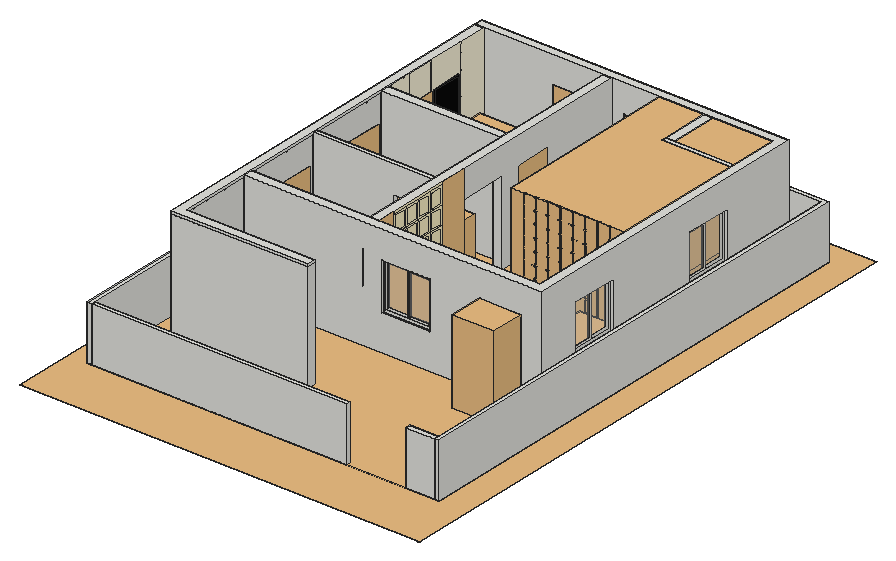
# SketchUp Ruby script. Lengths in inches.
U = 1.inch
M = Sketchup.active_model
def pt(a) = Geom::Point3d.new(a.map { |v| v * U })
def face(e, loops, mat)
  f = e.add_face(loops[0].map { |a| pt(a) })
  loops[1..].each { |l| e.add_face(l.map { |a| pt(a) }).erase! }
  f.material = f.back_material = mat if mat
  f
end
# faces: each face lists its corners as indices into pts; further lists are holes
def faces(e, pts, list, mat = nil) = list.each { |f| face(e, (f[0].is_a?(Array) ? f : [f]).map { |l| l.map { |i| pts[i] } }, mat) }
# xy, xz, yz: faces in a plane at the given z, y or x. An outline is a flat list of corners, or four numbers for a rectangle; further outlines are holes
def ring(l) = l.size == 4 ? [[l[0], l[1]], [l[2], l[1]], [l[2], l[3]], [l[0], l[3]]] : l.each_slice(2).to_a
def flat(e, list, mat, &to3) = list.each { |f| face(e, (f[0].is_a?(Array) ? f : [f]).map { |l| ring(l).map { |u, v| to3.(u, v) } }, mat) }
def xy(e, z, list, mat = nil) = flat(e, list, mat) { |x, y| [x, y, z] }
def xz(e, y, list, mat = nil) = flat(e, list, mat) { |x, z| [x, y, z] }
def yz(e, x, list, mat = nil) = flat(e, list, mat) { |y, z| [x, y, z] }
def lines(e, pts, list) = list.each { |a, b| e.add_line(pt(pts[a]), pt(pts[b])) }
# prism: a flat outline (further loops are holes) pulled along v
def prism(e, loops, v, mat = nil)
  f = face(e, loops, mat); d = Geom::Vector3d.new(v.map { |x| x * U })
  f.pushpull(f.normal.samedirection?(d) ? d.length : -d.length)
end
def box(e, o, s, mat = nil) = prism(e, [[o, [o[0] + s[0], o[1], o[2]], [o[0] + s[0], o[1] + s[1], o[2]], [o[0], o[1] + s[1], o[2]]]], [0, 0, s[2]], mat)
def at(x, y, z, deg = 0) = Geom::Transformation.translation(pt([x, y, z])) * Geom::Transformation.rotation(ORIGIN, Z_AXIS, deg.degrees)
def axes(o, x, y, z) = Geom::Transformation.new([*x, 0, *y, 0, *z, 0, *pt(o).to_a, 1])
def part(name) = M.definitions.add(name)
# library, detail: a bought-in or finely detailed component or shape, given as its bounding box
def library(name, o, s) = part(name).tap { |d| box(d.entities, o, s) }
def detail(e, o, s) = box(e.add_group.entities, o, s)
def put(e, d, t, mat = nil) = e.add_instance(d, t).tap { |i| i.material = mat if mat }
def group(e, t, mat = nil) = e.add_group.tap { |g| g.transformation = t; g.material = mat if mat }.entities
root = M.entities
M.materials.add("0939 AP 7866 BUTTER SCOTCH").color = [249, 239, 196]
M.materials.add("0949 AP 7872 SAFFRON SMILE").color = [254, 228, 149]
M.materials.add("0976 AP 9885 Military Boots-N").color = [124, 94, 57]
M.materials.add("0977 AP 7900 CANDLE LIGHT").color = [247, 240, 215]
M.materials.add("CLC2-EXTRACTOR-Cristal placa").color = [10, 10, 10]
M.materials.add("Cattelan Italy Adam 3").color = [207, 207, 207]
M.materials.add("[Color M00]").color = [255, 255, 255]
M.materials.add("[Color M09]").color = [0, 0, 0]
M.materials.add("[CoolGray4]").color = [225, 226, 230]
M.materials["[CoolGray4]"].alpha = 0.26
M.materials.add("[Translucent Glass Gray]").color = [128, 128, 128]
M.materials["[Translucent Glass Gray]"].alpha = 0.5
M.materials.add("[Translucent Glass Tinted]1").color = [7, 201, 240]
M.materials["[Translucent Glass Tinted]1"].alpha = 0.48
M.materials.add("[Wood Cherry Original]").color = [152, 86, 42]
M.materials.add("[Wood Floor Parquet]").color = [145, 89, 39]
M.materials.add("[Wood Veneer 02]").color = [190, 128, 91]
c1 = library("FLOOPLAN+DWG.dwg",[0,0,0],[402.1875,574.41,0.01])
c2 = part("Window sash")
g1 = group(c2.entities,at(0.98,0,0))
prism(g1,[[[-0.98,0,0],[30.98,0,0],[30.98,0,45.6],[-0.98,0,45.6]],[[29.01,0,43.625],[29.01,0,1.97],[0.98,0,1.97],[0.98,0,43.625]]],[0,1.18,0])
g2 = group(c2.entities,at(1.97,0.59,1.97))
xz(g2,0,[[0,0,28.03,41.66]],"[CoolGray4]")
c3 = part("Sliding window")
put(c3.entities,c2,at(31.97,2.82,1.97))
put(c3.entities,c2,at(1.97,1.25,1.97))
g3 = group(c3.entities,at(0,0,0))
prism(g3,[[[65.9,4.72,0],[0,4.72,0],[0,4.72,49.53],[65.9,4.72,49.53]],[[1.97,4.72,47.5625],[1.97,4.72,1.97],[63.93,4.72,1.97],[63.93,4.72,47.5625]]],[0,-4.72,0])
c4 = part("ventilator")
g4 = group(c4.entities,at(0,0,0))
xy(g4,0,[[0,0,24,1],[0,1,24,6.83]],"[Wood Floor Parquet]")
xy(g4,1.75,[[2,0,22,6.83]],"[Wood Floor Parquet]")
xy(g4,21.87,[[2,0,22,6.83]],"[Wood Cherry Original]")
xy(g4,23.62,[[0,0,24,1],[0,1,24,6.83]],"[Wood Floor Parquet]")
xz(g4,0,[[[0,0,24,23.62],[2,1.75,22,21.87]]],"[Wood Floor Parquet]")
xz(g4,6.83,[[[0,0,24,23.62],[2,1.75,22,21.87]]],"[Wood Cherry Original]")
yz(g4,0,[[0,0,1,23.62],[1,0,6.83,23.62]],"[Wood Floor Parquet]")
yz(g4,2,[[0,1.75,6.83,1.75,6.83,7.66,0,3.5],[0,3.5,6.83,7.66,6.83,11.8125,0,7.66],[0,7.66,6.83,11.8125,6.83,15.97,0,11.8125],[0,11.8125,6.83,15.97,6.83,20.12,0,15.97],[0,15.97,6.83,20.12,6.83,21.87,0,21.87]],"[Wood Floor Parquet]")
yz(g4,22,[[0,1.75,0,3.5,6.83,7.66,6.83,1.75],[0,3.5,0,7.66,6.83,11.8125,6.83,7.66],[0,7.66,0,11.8125,6.83,15.97,6.83,11.8125],[0,11.8125,0,15.97,6.83,20.12,6.83,15.97],[0,15.97,0,21.87,6.83,21.87,6.83,20.12]],"[Wood Floor Parquet]")
yz(g4,24,[[0,0,1,23.62],[1,0,6.83,23.62]],"[Wood Floor Parquet]")
p = [[2,0,3.5],[2,6.83,7.66],[22,6.83,7.66],[22,0,3.5],[2,6.83,11.8125],[2,0,7.66],
  [22,0,7.66],[22,6.83,11.8125],[2,0,11.8125],[2,6.83,15.97],[22,6.83,15.97],[22,0,11.8125],
  [2,6.83,20.12],[2,0,15.97],[22,0,15.97],[22,6.83,20.12]]
faces(g4,p,[[0,1,2,3],[4,5,6,7],[8,9,10,11]],"[Translucent Glass Tinted]1")
faces(g4,p,[[12,13,14,15]],"[Translucent Glass Gray]")
c5 = library("door by lz",[5.91,-4.92,0],[35.43,6.61,78.74])
c6 = library("Open hinged door",[0,0,0],[71.65,72.83,104.72])
c7 = library("Wall hung toilet",[0.42,0,0],[26.94,19.69,42.125])
c8 = library("3D DOOR",[-0.52,0,0],[35.44,5.29,86.61])
c9 = library("DINING SET",[25.27,8.07,0],[68.7,94.48,53.71])
c10 = library("Спалня Венид",[0.07,-0.07,0],[84.71,86.8,39])
c11 = library("window curtain",[0,0,0],[144.39,2.04,43.18])
c12 = library("sofaD71839)",[0.35,-39.08,0.31],[80.46,34.29,30.24])
c13 = library("Layer_AVLA\#1",[-10.99,-0.19,-10.42],[21.98,0.74,15.78])
c14 = part("Group12\#1")
xy(c14.entities,0,[[329.9,217.87,329.9,226.87,341.6,226.87,341.6,519.37,41.6,519.37,41.6,528.37,350.6,528.37,350.6,217.87],[50.6,217.87,287.9,226.87]])
xy(c14.entities,36,[[189.83,217.87,237.83,226.87],[341.6,260,350.6,308],[341.6,403.49,350.6,451.49]])
xy(c14.entities,48,[[123.82,519.37,159.82,528.37]])
xy(c14.entities,60,[[192.32,519.37,216.32,528.37],[300.77,519.37,324.77,528.37]])
xy(c14.entities,84,[[189.83,217.87,237.83,226.87],[287.9,217.87,329.9,226.87],[341.6,260,350.6,308],[341.6,403.49,350.6,451.49],[123.82,519.37,159.82,528.37],
  [192.32,519.37,216.32,528.37],[300.77,519.37,324.77,528.37]])
xy(c14.entities,112,[[50.6,217.87,350.6,217.87,350.6,528.37,41.6,528.37,41.6,519.37,341.6,519.37,341.6,226.87,50.6,226.87]])
xz(c14.entities,217.87,[[[50.6,0,287.9,0,287.9,84,329.9,84,329.9,0,350.6,0,350.6,112,50.6,112],[189.83,36,237.83,84]]])
xz(c14.entities,226.87,[[[50.6,0,50.6,112,341.6,112,341.6,0,329.9,0,329.9,84,287.9,84,287.9,0],[189.83,36,237.83,84]]])
xz(c14.entities,260,[[341.6,36,350.6,84]])
xz(c14.entities,308,[[341.6,36,350.6,84]])
xz(c14.entities,403.49,[[341.6,36,350.6,84]])
xz(c14.entities,451.49,[[341.6,36,350.6,84]])
xz(c14.entities,519.37,[[[41.6,0,341.6,112],[123.82,48,159.82,84],[192.32,60,216.32,84],[300.77,60,324.77,84]]])
xz(c14.entities,528.37,[[[41.6,0,350.6,112],[123.82,48,159.82,84],[192.32,60,216.32,84],[300.77,60,324.77,84]]])
yz(c14.entities,41.6,[[519.37,0,528.37,112]])
yz(c14.entities,50.6,[[217.87,0,226.87,112]])
yz(c14.entities,123.82,[[519.37,48,528.37,84]])
yz(c14.entities,159.82,[[519.37,48,528.37,84]])
yz(c14.entities,189.83,[[217.87,36,226.87,84]])
yz(c14.entities,192.32,[[519.37,60,528.37,84]])
yz(c14.entities,216.32,[[519.37,60,528.37,84]])
yz(c14.entities,237.83,[[217.87,36,226.87,84]])
yz(c14.entities,287.9,[[217.87,0,226.87,84]])
yz(c14.entities,300.77,[[519.37,60,528.37,84]])
yz(c14.entities,324.77,[[519.37,60,528.37,84]])
yz(c14.entities,329.9,[[217.87,0,226.87,84]])
yz(c14.entities,341.6,[[[226.87,0,519.37,112],[260,36,308,84],[403.49,36,451.49,84]]])
yz(c14.entities,350.6,[[[217.87,0,528.37,112],[260,36,308,84],[403.49,36,451.49,84]]])
c15 = part("Group13\#1")
xy(c15.entities,0,[[41.6,136.87,41.6,519.37,50.6,519.37,50.6,491.06,51.07,491.06,51.07,490.59,50.6,490.59,50.6,145.87,179.6,145.87,179.6,136.87],[50.6,399.37,51.07,452.7],[50.6,452.7,51.07,453.17],[50.6,453.17,51.07,490.59],[50.6,491.06,51.07,519.37]])
xy(c15.entities,36,[[41.6,250.14,50.6,298.14],[41.6,336.36,50.6,384.36],[41.6,403.49,50.6,451.49],[50.6,403.49,51.07,451.49]])
xy(c15.entities,84,[[41.6,250.14,50.6,298.14],[41.6,336.36,50.6,384.36],[41.6,403.49,50.6,451.49],[50.6,403.49,51.07,451.49]])
xy(c15.entities,109.4375,[[41.6,136.87,41.6,519.37,50.6,519.37,50.6,145.87,179.6,145.87,179.6,136.87]])
xy(c15.entities,112,[[41.6,136.87,179.6,136.87,179.6,145.87,50.6,145.87,50.6,519.37,41.6,519.37],[50.6,399.37,51.07,452.7],[50.6,452.7,51.07,453.17],[50.6,453.17,51.07,490.59],[50.6,490.59,51.07,491.06],
  [50.6,491.06,51.07,519.37]])
xz(c15.entities,136.87,[[41.6,0,179.6,109.4375],[41.6,109.4375,179.6,112]])
xz(c15.entities,145.87,[[50.6,0,179.6,109.4375],[50.6,109.4375,179.6,112]])
xz(c15.entities,250.14,[[41.6,36,50.6,84]])
xz(c15.entities,298.14,[[41.6,36,50.6,84]])
xz(c15.entities,336.36,[[41.6,36,50.6,84]])
xz(c15.entities,384.36,[[41.6,36,50.6,84]])
xz(c15.entities,399.37,[[50.6,0,51.07,112]])
xz(c15.entities,403.49,[[41.6,36,50.6,84],[50.6,36,51.07,84]])
xz(c15.entities,451.49,[[41.6,36,50.6,84],[50.6,36,51.07,84]])
xz(c15.entities,452.7,[[50.6,0,51.07,112]])
xz(c15.entities,453.17,[[50.6,0,51.07,112]])
xz(c15.entities,490.59,[[50.6,0,51.07,109.4375],[50.6,109.4375,51.07,112]])
xz(c15.entities,491.06,[[50.6,0,51.07,109.4375],[50.6,109.4375,51.07,112]])
xz(c15.entities,519.37,[[41.6,0,50.6,109.4375],[50.6,0,51.07,112],[41.6,109.4375,50.6,112]])
yz(c15.entities,41.6,[[[136.87,0,519.37,109.4375],[250.14,36,298.14,84],[336.36,36,384.36,84],[403.49,36,451.49,84]],[136.87,109.4375,519.37,112]])
yz(c15.entities,50.6,[[[145.87,0,399.37,109.4375],[250.14,36,298.14,84],[336.36,36,384.36,84]],[[399.37,0,452.7,109.4375],[403.49,36,451.49,84]],[452.7,0,453.17,109.4375],[453.17,0,490.59,109.4375],[491.06,0,519.37,109.4375],
  [145.87,109.4375,399.37,112],[399.37,109.4375,452.7,112],[452.7,109.4375,453.17,112],[453.17,109.4375,490.59,112],[490.59,109.4375,491.06,112],
  [491.06,109.4375,519.37,112]])
yz(c15.entities,51.07,[[427.02,0,427.49,36],[452.7,0,453.17,112],[490.59,0,491.06,112],[425.5625,84,426.04,112]],"0976 AP 9885 Military Boots-N")
yz(c15.entities,51.07,[[399.37,0,427.02,0,427.02,36,403.49,36,403.49,84,425.5625,84,425.5625,112,399.37,112],[427.49,0,452.7,0,452.7,112,426.04,112,426.04,84,451.49,84,451.49,36,427.49,36],[453.17,0,490.59,112],[491.06,0,519.37,112]],"0977 AP 7900 CANDLE LIGHT")
yz(c15.entities,179.6,[[136.87,0,145.87,109.4375],[136.87,109.4375,145.87,112]])
c16 = library("Group621\#1",[-13.47,-47,0],[26.94,94,0.5])
c17 = library("Group691\#2",[-8.65,-47,0],[17.3,94,0.5])
c18 = part("Group14\#1")
xy(c18.entities,0,[[170.6,226.87,179.6,333.37],[170.6,381.37,179.6,402.37],[170.6,438.37,179.6,519.37]])
xy(c18.entities,84,[[170.6,333.37,179.6,381.37],[170.6,402.37,179.6,438.37]])
xy(c18.entities,112,[[170.6,226.87,179.6,519.37]])
xz(c18.entities,226.87,[[170.6,0,179.6,112]])
xz(c18.entities,333.37,[[170.6,0,179.6,84]])
xz(c18.entities,381.37,[[170.6,0,179.6,84]])
xz(c18.entities,402.37,[[170.6,0,179.6,84]])
xz(c18.entities,438.37,[[170.6,0,179.6,84]])
xz(c18.entities,519.37,[[170.6,0,179.6,112]])
yz(c18.entities,170.6,[[226.87,0,226.87,112,519.37,112,519.37,0,438.37,0,438.37,84,402.37,84,402.37,0,381.37,0,381.37,84,333.37,84,333.37,0]])
yz(c18.entities,179.6,[[226.87,0,333.37,18],[381.37,0,402.37,0,402.37,84,438.37,84,438.37,0,519.37,0,519.37,112,333.37,112,333.37,84,381.37,84],[244.16,18,244.87,112]])
yz(c18.entities,179.6,[[244.87,18,306.43,112]],"0939 AP 7866 BUTTER SCOTCH")
put(c18.entities,c16,axes([179.6,319.76,65],[0,1,0],[0,0,1],[1,0,0]),"0939 AP 7866 BUTTER SCOTCH")
put(c18.entities,c17,axes([179.6,235.52,65],[0,1,0],[0,0,1],[1,0,0]),"0939 AP 7866 BUTTER SCOTCH")
c19 = part("Group15\#1")
box(c19.entities,[50.6,390.37,0],[120,9,112])
c20 = library("Group16\#1",[227.6,332.87,0],[114,186.5,112])
c21 = part("Group17\#1")
box(c21.entities,[272.6,471.37,0],[9,48,112])
c22 = part("Group18\#1")
prism(c22.entities,[[[341.6,471.37,0],[338.6,471.37,0],[338.6,471.37,84],[312.6,471.37,84],[312.6,471.37,0],[272.6,471.37,0],[272.6,471.37,112],[341.6,471.37,112]]],[0,-4.5,0])
c23 = part("Group19\#1")
prism(c23.entities,[[[170.6,309.37,0],[167.6,309.37,0],[167.6,309.37,84],[131.6,309.37,84],[131.6,309.37,0],[50.6,309.37,0],[50.6,309.37,112],[170.6,309.37,112]]],[0,-4.5,0])
c24 = part("Group26\#1")
box(c24.entities,[340.13,60.37,0],[28.47,4.5,54.875])
c25 = part("Group24\#1")
prism(c25.entities,[[[368.6,546.37,0],[23.6,546.37,0],[23.6,60.37,0],[19.1,60.37,0],[19.1,550.87,0],[373.1,550.87,0],[373.1,60.37,0],[368.6,60.37,0]]],[0,0,54.875])
put(c25.entities,c24,at(0,0,0))
c26 = part("Group25\#1")
box(c26.entities,[23.6,60.37,0],[256.53,4.5,54.875])
c27 = library("Group\#12",[0,-0.0625,0],[48,15.0625,24])
c28 = library("Group\#13",[0,-0.13,0],[120,18.13,42.48])
c29 = library("Group\#14",[0,-8.89,-5.43],[120,21.66,33.43])
c30 = part("Group\#15")
prism(c30.entities,[[[1.2,0.71,0],[0.83,0.71,0.03],[0.53,0.71,0.13],[0.3,0.71,0.3],[0.13,0.71,0.53],[0.03,0.71,0.83],[0,0.71,1.2],[0,0.71,10.8],[0.03,0.71,11.17],[0.13,0.71,11.47],[0.3,0.71,11.7],[0.53,0.71,11.87],[0.83,0.71,11.97],[1.2,0.71,12],[10.8,0.71,12],[11.17,0.71,11.97],[11.47,0.71,11.87],[11.7,0.71,11.7],[11.87,0.71,11.47],[11.97,0.71,11.17],[12,0.71,10.8],[12,0.71,1.2],[11.97,0.71,0.83],[11.87,0.71,0.53],[11.7,0.71,0.3],[11.47,0.71,0.13],[11.17,0.71,0.03],[10.8,0.71,0]]],[0,-0.39,0])
c31 = part("Group\#17")
xy(c31.entities,0,[[0,0,0.47,15]])
xy(c31.entities,1.35,[[0.24,1.82,0.47,13.18]])
xy(c31.entities,16.65,[[0.24,1.82,0.47,13.18]])
xy(c31.entities,18,[[0,0,0.47,15]])
xz(c31.entities,0,[[0,0,0.47,18]])
xz(c31.entities,1.35,[[0.24,1.82,0.47,16.18]])
xz(c31.entities,13.65,[[0.24,1.82,0.47,16.18]])
xz(c31.entities,15,[[0,0,0.47,18]])
yz(c31.entities,0,[[0,0,15,18]])
yz(c31.entities,0.24,[[1.82,1.35,13.18,1.35,13.33,1.36,13.44,1.4,13.54,1.46,13.6,1.56,13.64,1.67,13.65,1.82,13.65,16.18,13.64,16.33,13.6,16.44,13.54,16.54,13.44,16.6,13.33,16.64,13.18,16.65,1.82,16.65,1.67,16.64,1.56,16.6,1.46,16.54,1.4,16.44,1.36,16.33,1.35,16.18,1.35,1.82,1.36,1.67,1.4,1.56,1.46,1.46,1.56,1.4,1.67,1.36]])
yz(c31.entities,0.47,[[[0,0,15,18],[1.82,1.35,1.67,1.36,1.56,1.4,1.46,1.46,1.4,1.56,1.36,1.67,1.35,1.82,1.35,16.18,1.36,16.33,1.4,16.44,1.46,16.54,1.56,16.6,1.67,16.64,1.82,16.65,13.18,16.65,13.33,16.64,13.44,16.6,13.54,16.54,13.6,16.44,13.64,16.33,13.65,16.18,13.65,1.82,13.64,1.67,13.6,1.56,13.54,1.46,13.44,1.4,13.33,1.36,13.18,1.35]]])
p = [[0.47,1.82,1.35],[0.24,1.82,1.35],[0.24,1.67,1.36],[0.47,1.67,1.36],[0.47,13.33,1.36],[0.24,13.33,1.36],
  [0.24,13.18,1.35],[0.47,13.18,1.35],[0.47,1.56,1.4],[0.24,1.56,1.4],[0.24,1.46,1.46],[0.47,1.46,1.46],
  [0.47,13.44,1.4],[0.24,13.44,1.4],[0.47,13.54,1.46],[0.24,13.54,1.46],[0.24,1.4,1.56],[0.47,1.4,1.56],
  [0.47,13.6,1.56],[0.24,13.6,1.56],[0.24,1.36,1.67],[0.47,1.36,1.67],[0.47,13.64,1.67],[0.24,13.64,1.67],
  [0.24,1.35,1.82],[0.47,1.35,1.82],[0.47,13.65,1.82],[0.24,13.65,1.82],[0.24,1.36,16.33],[0.47,1.36,16.33],
  [0.47,1.35,16.18],[0.24,1.35,16.18],[0.47,13.64,16.33],[0.24,13.64,16.33],[0.24,13.65,16.18],[0.47,13.65,16.18],
  [0.24,1.4,16.44],[0.47,1.4,16.44],[0.47,13.6,16.44],[0.24,13.6,16.44],[0.24,1.46,16.54],[0.47,1.46,16.54],
  [0.47,13.54,16.54],[0.24,13.54,16.54],[0.24,1.56,16.6],[0.47,1.56,16.6],[0.47,13.44,16.6],[0.24,13.44,16.6],
  [0.24,1.67,16.64],[0.47,1.67,16.64],[0.24,1.82,16.65],[0.47,1.82,16.65],[0.47,13.18,16.65],[0.24,13.18,16.65],
  [0.24,13.33,16.64],[0.47,13.33,16.64]]
faces(c31.entities,p,[[0,1,2,3],[4,5,6,7],[8,9,10,11],[3,2,9,8],[12,13,5,4],[14,15,13,12],[11,10,16,17],[18,19,15,14],
  [17,16,20,21],[22,23,19,18],[21,20,24,25],[26,27,23,22],[28,29,30,31],[32,33,34,35],[36,37,29,28],[38,39,33,32],
  [40,41,37,36],[42,43,39,38],[44,45,41,40],[46,47,43,42],[48,49,45,44],[50,51,49,48],[52,53,54,55],[55,54,47,46]])
detail(root,[255.5,283.71,55.12],[29,0.2,29.01])
put(root,c1,at(-19.1,-60.37,0))
put(root,c3,axes([26.37,343.12,36],[0,0.72837,0],[0.59,0,0],[0,0,0.96906]))
put(root,c3,axes([26.37,275.99,36],[0,0.72837,0],[0.59,0,0],[0,0,0.96906]))
put(root,c3,axes([26.98,189.77,36],[0,0.72837,0],[0.59,0,0],[0,0,0.96906]))
put(root,c3,axes([328.34,343.12,36],[0,0.72837,0],[-0.59,0,0],[0,0,0.96906]))
put(root,c3,axes([328.34,199.625,36],[0,0.72837,0],[-0.59,0,0],[0,0,0.96906]))
put(root,c3,axes([104.72,464.63,48],[0.54627,0,0],[0,-0.3068,0],[0,0,0.7268]))
put(root,c4,axes([173.22,459.04,60],[1,0,0],[0,1,0],[0,0,1.016]))
put(root,c4,axes([281.67,459.04,60],[1,0,0],[0,1,0],[0,0,1.016]))
put(root,c3,axes([218.74,160.2,36],[-0.72837,0,0],[0,0.59,0],[0,0,0.96906]))
put(root,c5,axes([158.8125,384.01,0],[0,-1.016,0],[1,0,0],[0,0,1.07]))
put(root,c5,axes([215.08,327.01,0],[0,-1.016,0],[1,0,0],[0,0,1.07]))
put(root,c6,axes([268.8,123.04,0],[0.58615,0,0],[0,0.5874,0],[0,0,0.80211]))
put(root,c7,at(262.5,451.65,2,-90))
put(root,c8,axes([293.88,405.89,0],[0.73378,0,0],[0,1,0],[0,0,0.97]))
put(root,c9,axes([140.2,238.87,-5.99],[0,0.87,0],[-0.87,0,0],[0,0,0.87]))
put(root,c10,axes([227.125,372.21,0],[1,0,0],[0,-1,0],[0,0,1]))
put(root,c11,axes([320.47,391.61,40.82],[0,-0.34247,0],[1,0,0],[0,0,1.02]))
put(root,c12,at(323.14,265.07,0,-90))
put(root,c10,axes([120.73,452.05,0],[0,-1,0],[-1,0,0],[0,0,1]))
put(root,c13,axes([33.07,366.5,67.38],[0,2.30992,0],[-2,0,0],[0,0,3.10311]))
put(root,c13,axes([32.59,299.68,67.38],[0,2.30992,0],[-2,0,0],[0,0,3.10311]),"[Color M00]")
put(root,c13,axes([32.59,213.49,67.38],[0,2.30992,0],[-2,0,0],[0,0,3.10311]))
put(root,c13,axes([122.41,457.91,72.16],[1.8174,0,0],[0,2,0],[0,0,2.53214]))
put(root,c13,axes([196.12,167.59,69.4375],[2.30992,0,0],[0,-2,0],[0,0,3.10311]))
put(root,c14,at(-19.1,-60.37,0))
put(root,c15,at(-19.1,-60.37,0))
put(root,c18,at(-19.1,-60.37,0))
put(root,c19,at(-19.1,-60.37,0))
put(root,c20,at(-19.1,-60.37,0),"Cattelan Italy Adam 3")
put(root,c21,at(-19.1,-60.37,0))
put(root,c22,at(-19.1,-60.37,0))
put(root,c23,at(-19.1,-60.37,0))
g5 = group(root,at(0,0,-6))
box(g5,[0,0,0],[354,490.5,6])
put(root,c25,at(-19.1,-60.37,0))
put(root,c26,at(-19.1,-60.37,0))
g6 = group(root,at(321.52,309.65,36),"[Color M09]")
xy(g6,0,[[0,0,0.98,30.16]])
xy(g6,48,[[0,0,0.98,30.16]])
xz(g6,0,[[0,0,0.98,48]])
xz(g6,30.16,[[0,0,0.98,48]])
yz(g6,0,[[[0,0,30.16,48],[0.71,0.71,29.45,47.29]],[0.71,0.71,29.45,47.29]])
yz(g6,0.98,[[0,0,30.16,48]])
put(root,c27,at(160.5,444,6))
put(root,c28,at(31.5,166.5,0))
put(root,c29,at(31.5,166.5,59),"0949 AP 7872 SAFFRON SMILE")
put(root,c30,at(220.97,272.29,100))
put(root,c30,at(233.44,272.29,100))
put(root,c30,at(245.92,272.29,100))
put(root,c30,at(258.39,272.29,100))
put(root,c30,at(270.86,272.29,100))
put(root,c30,at(283.33,272.29,100))
put(root,c30,at(295.81,272.29,100))
put(root,c30,at(220.97,272.29,87.53))
put(root,c30,at(233.44,272.29,87.53))
put(root,c30,at(245.92,272.29,87.53))
put(root,c30,at(270.86,272.29,87.53))
put(root,c30,at(283.33,272.29,87.53))
put(root,c30,at(295.81,272.29,87.53))
put(root,c30,at(258.39,272.29,87.53))
put(root,c30,at(221.04,272.29,75.06))
put(root,c30,at(233.51,272.29,75.06))
put(root,c30,at(245.98,272.29,75.06))
put(root,c30,at(270.93,272.29,75.06))
put(root,c30,at(283.4,272.29,75.06))
put(root,c30,at(295.875,272.29,75.06))
put(root,c30,at(258.46,272.29,75.06))
put(root,c30,at(220.97,272.29,62.58))
put(root,c30,at(233.44,272.29,62.58))
put(root,c30,at(245.92,272.29,62.58))
put(root,c30,at(270.86,272.29,62.58))
put(root,c30,at(283.33,272.29,62.58))
put(root,c30,at(295.81,272.29,62.58))
put(root,c30,at(258.39,272.29,62.58))
put(root,c30,at(220.97,272.29,50.45))
put(root,c30,at(233.44,272.29,50.45))
put(root,c30,at(245.92,272.29,50.45))
put(root,c30,at(270.86,272.29,50.45))
put(root,c30,at(283.33,272.29,50.45))
put(root,c30,at(295.81,272.29,50.45))
put(root,c30,at(258.39,272.29,50.45))
put(root,c30,at(220.97,272.29,37.94))
put(root,c30,at(233.44,272.29,37.94))
put(root,c30,at(245.92,272.29,37.94))
put(root,c30,at(270.86,272.29,37.94))
put(root,c30,at(283.33,272.29,37.94))
put(root,c30,at(295.81,272.29,37.94))
put(root,c30,at(258.39,272.29,37.94))
put(root,c30,at(220.97,272.29,25.17))
put(root,c30,at(233.44,272.29,25.17))
put(root,c30,at(245.92,272.29,25.17))
put(root,c30,at(270.86,272.29,25.17))
put(root,c30,at(283.33,272.29,25.17))
put(root,c30,at(295.81,272.29,25.17))
put(root,c30,at(258.39,272.29,25.17))
put(root,c30,at(220.97,272.29,12.59))
put(root,c30,at(233.44,272.29,12.59))
put(root,c30,at(245.92,272.29,12.59))
put(root,c30,at(270.86,272.29,12.59))
put(root,c30,at(283.33,272.29,12.59))
put(root,c30,at(295.81,272.29,12.59))
put(root,c30,at(258.39,272.29,12.59))
put(root,c30,at(220.97,272.29,0.22))
put(root,c30,at(233.44,272.29,0.22))
put(root,c30,at(245.92,272.29,0.22))
put(root,c30,at(270.86,272.29,0.22))
put(root,c30,at(283.33,272.29,0.22))
put(root,c30,at(295.81,272.29,0.22))
put(root,c30,at(258.39,272.29,0.22))
g7 = group(root,at(160.5,166.5,6),"0939 AP 7866 BUTTER SCOTCH")
xy(g7,0,[[0,0,13,106.5]])
xy(g7,0.47,[[12.29,0.47,13,0.59],[12.29,0.59,13,35.54],[12.29,35.54,13,35.66],[12.29,70.84,13,106.03]])
xy(g7,0.47,[[12.29,35.66,13,70.84]],"0939 AP 7866 BUTTER SCOTCH")
xy(g7,0.59,[[12.29,0.59,13,35.54],[12.29,70.96,13,105.91]])
xy(g7,0.94,[[1,36.13,12.29,70.37]],"[Wood Veneer 02]")
xy(g7,11.06,[[1,36.13,12.29,70.37]],"[Wood Veneer 02]")
xy(g7,11.41,[[12.29,0.59,13,35.54],[12.29,70.96,13,105.91]])
xy(g7,11.53,[[12.29,0.47,13,35.54],[12.29,35.54,13,35.66],[12.29,70.84,13,106.03]])
xy(g7,11.53,[[12.29,35.66,13,70.84]],"0939 AP 7866 BUTTER SCOTCH")
xy(g7,12,[[0,0,13,106.5]])
xz(g7,0,[[0,0,13,12]])
xz(g7,0.47,[[12.29,0.47,13,11.41],[12.29,11.41,13,11.53]])
xz(g7,0.59,[[12.29,0.59,13,11.41]])
xz(g7,35.54,[[12.29,0.59,13,11.41]])
xz(g7,36.13,[[1,0.94,12.29,11.06]],"[Wood Veneer 02]")
xz(g7,70.37,[[1,0.94,12.29,11.06]],"[Wood Veneer 02]")
xz(g7,70.96,[[12.29,0.59,13,11.41]])
xz(g7,105.91,[[12.29,0.59,13,11.41]])
xz(g7,106.03,[[12.29,0.47,13,11.53]])
xz(g7,106.5,[[0,0,13,12]])
yz(g7,0,[[0,0,106.5,12]])
yz(g7,1,[[36.13,0.94,70.37,11.06]],"[Wood Veneer 02]")
yz(g7,12.29,[[0.47,0.47,0.59,11.41],[0.59,0.47,35.54,0.59],[35.54,0.47,35.66,11.53],[[70.84,0.47,106.03,11.53],[70.96,0.59,105.91,11.41]],[0.47,11.41,35.54,11.53]])
yz(g7,12.29,[[[35.66,0.47,70.84,11.53],[36.13,0.94,70.37,11.06]]],"0939 AP 7866 BUTTER SCOTCH")
yz(g7,13,[[[0,0,106.5,12],[0.47,0.47,106.03,11.53]],[0.59,0.59,35.54,11.41],[70.96,0.59,105.91,11.41]])
put(root,c31,at(160.5,184.5,91.65),"0939 AP 7866 BUTTER SCOTCH")
put(root,c31,at(160.5,199.74,91.65),"0939 AP 7866 BUTTER SCOTCH")
put(root,c31,at(160.5,214.97,91.65),"0939 AP 7866 BUTTER SCOTCH")
put(root,c31,at(160.5,230.21,91.65),"0939 AP 7866 BUTTER SCOTCH")
put(root,c31,at(160.5,230.21,73.42),"0939 AP 7866 BUTTER SCOTCH")
put(root,c31,at(160.5,199.74,73.42),"0939 AP 7866 BUTTER SCOTCH")
put(root,c31,at(160.5,214.97,73.42),"0939 AP 7866 BUTTER SCOTCH")
put(root,c31,at(160.5,184.5,73.42),"0939 AP 7866 BUTTER SCOTCH")
put(root,c31,at(160.5,230.21,55.18),"0939 AP 7866 BUTTER SCOTCH")
put(root,c31,at(160.5,199.74,55.18),"0939 AP 7866 BUTTER SCOTCH")
put(root,c31,at(160.5,214.97,55.18),"0939 AP 7866 BUTTER SCOTCH")
put(root,c31,at(160.5,184.5,55.18),"0939 AP 7866 BUTTER SCOTCH")
put(root,c31,at(160.5,230.21,36.94),"0939 AP 7866 BUTTER SCOTCH")
put(root,c31,at(160.5,199.74,36.94),"0939 AP 7866 BUTTER SCOTCH")
put(root,c31,at(160.5,214.97,36.94),"0939 AP 7866 BUTTER SCOTCH")
put(root,c31,at(160.5,184.5,36.94),"0939 AP 7866 BUTTER SCOTCH")
put(root,c31,at(160.5,230.21,18.71),"0939 AP 7866 BUTTER SCOTCH")
put(root,c31,at(160.5,199.74,18.71),"0939 AP 7866 BUTTER SCOTCH")
put(root,c31,at(160.5,214.97,18.71),"0939 AP 7866 BUTTER SCOTCH")
put(root,c31,at(160.5,184.5,18.71),"0939 AP 7866 BUTTER SCOTCH")
g8 = group(root,at(172.79,202.16,6.59),"[Color M09]")
xy(g8,0,[[0,0,0.47,35.19]])
xy(g8,0.47,[[0,0.47,0.47,34.71]])
xy(g8,10.35,[[0,0.47,0.47,34.71]])
xy(g8,10.82,[[0,0,0.47,35.19]])
xz(g8,0,[[0,0,0.47,10.82]])
xz(g8,0.47,[[0,0.47,0.47,10.35]])
xz(g8,34.71,[[0,0.47,0.47,10.35]])
xz(g8,35.19,[[0,0,0.47,10.82]])
yz(g8,0,[[[0,0,35.19,10.82],[0.47,0.47,34.71,10.35]]])
yz(g8,0,[[0.47,0.47,34.71,10.35]],"[Translucent Glass Gray]")
yz(g8,0.47,[[[0,0,35.19,10.82],[0.47,0.47,34.71,10.35]]])
g9 = group(root,at(161.04,195.53,31.68),"[Color M09]")
box(g9,[0,0,0],[1.14,38.03,27.72])
g10 = group(root,at(31.97,395.55,40.47),"CLC2-EXTRACTOR-Cristal placa")
xy(g10,0,[[0,0,0.79,31.16]])
xy(g10,43.95,[[0,0,0.79,31.16]])
xz(g10,0,[[0,0,0.79,43.95]])
xz(g10,31.16,[[0,0,0.79,43.95]])
yz(g10,0,[[0,0,31.16,43.95]])
yz(g10,0.79,[[[0,0,31.16,43.95],[0.71,0.71,30.45,43.24]],[0.71,0.71,30.45,43.24]])
